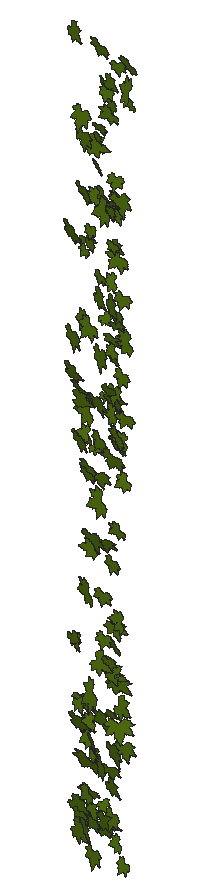
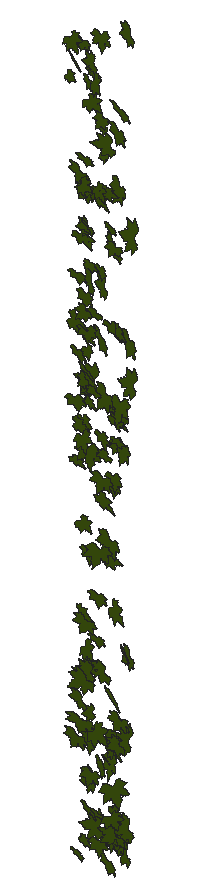
# SketchUp Ruby script. Lengths in inches.
U = 1.inch
M = Sketchup.active_model
def pt(a) = Geom::Point3d.new(a.map { |v| v * U })
def face(e, loops, mat)
  f = e.add_face(loops[0].map { |a| pt(a) })
  loops[1..].each { |l| e.add_face(l.map { |a| pt(a) }).erase! }
  f.material = f.back_material = mat if mat
  f
end
# faces: each face lists its corners as indices into pts; further lists are holes
def faces(e, pts, list, mat = nil) = list.each { |f| face(e, (f[0].is_a?(Array) ? f : [f]).map { |l| l.map { |i| pts[i] } }, mat) }
# xy, xz, yz: faces in a plane at the given z, y or x. An outline is a flat list of corners, or four numbers for a rectangle; further outlines are holes
def ring(l) = l.size == 4 ? [[l[0], l[1]], [l[2], l[1]], [l[2], l[3]], [l[0], l[3]]] : l.each_slice(2).to_a
def flat(e, list, mat, &to3) = list.each { |f| face(e, (f[0].is_a?(Array) ? f : [f]).map { |l| ring(l).map { |u, v| to3.(u, v) } }, mat) }
def xy(e, z, list, mat = nil) = flat(e, list, mat) { |x, y| [x, y, z] }
def xz(e, y, list, mat = nil) = flat(e, list, mat) { |x, z| [x, y, z] }
def yz(e, x, list, mat = nil) = flat(e, list, mat) { |y, z| [x, y, z] }
def lines(e, pts, list) = list.each { |a, b| e.add_line(pt(pts[a]), pt(pts[b])) }
# prism: a flat outline (further loops are holes) pulled along v
def prism(e, loops, v, mat = nil)
  f = face(e, loops, mat); d = Geom::Vector3d.new(v.map { |x| x * U })
  f.pushpull(f.normal.samedirection?(d) ? d.length : -d.length)
end
def box(e, o, s, mat = nil) = prism(e, [[o, [o[0] + s[0], o[1], o[2]], [o[0] + s[0], o[1] + s[1], o[2]], [o[0], o[1] + s[1], o[2]]]], [0, 0, s[2]], mat)
def at(x, y, z, deg = 0) = Geom::Transformation.translation(pt([x, y, z])) * Geom::Transformation.rotation(ORIGIN, Z_AXIS, deg.degrees)
def axes(o, x, y, z) = Geom::Transformation.new([*x, 0, *y, 0, *z, 0, *pt(o).to_a, 1])
def part(name) = M.definitions.add(name)
# library, detail: a bought-in or finely detailed component or shape, given as its bounding box
def library(name, o, s) = part(name).tap { |d| box(d.entities, o, s) }
def detail(e, o, s) = box(e.add_group.entities, o, s)
def put(e, d, t, mat = nil) = e.add_instance(d, t).tap { |i| i.material = mat if mat }
def group(e, t, mat = nil) = e.add_group.tap { |g| g.transformation = t; g.material = mat if mat }.entities
root = M.entities
M.materials.add("[Vegetation Blur 03]").color = [83, 114, 18]
c1 = part("ivy")
xy(c1.entities,0,[[0.782,0,0.786,0,0.787,0.005,0.789,0.009,0.821,0.072,0.875,0.147,1.001,0.272,1.073,0.331,1.137,0.363,1.178,0.379,1.223,0.384,1.272,0.383,1.311,0.374,1.36,0.355,1.399,0.334,1.491,0.285,1.541,0.244,1.583,0.199,1.617,0.15,1.64,0.128,1.662,0.115,1.717,0.105,1.745,0.093,1.784,0.054,1.819,0.057,1.854,0.064,1.882,0.075,1.896,0.074,1.91,0.071,1.937,0.063,1.964,0.053,1.99,0.038,2.016,0.015,2.034,0.002,2.04,0,2.038,0.003,2.036,0.007,2.033,0.038,2.036,0.068,2.045,0.1,2.055,0.116,2.064,0.123,2.077,0.129,2.088,0.129,2.106,0.132,2.118,0.13,2.179,0.132,2.207,0.133,2.225,0.133,2.242,0.138,2.22,0.162,2.207,0.186,2.206,0.213,2.212,0.236,2.228,0.262,2.247,0.274,2.298,0.283,2.355,0.294,2.37,0.296,2.376,0.295,2.377,0.3,2.377,0.303,2.385,0.329,2.411,0.37,2.426,0.392,2.449,0.407,2.511,0.426,2.561,0.444,2.619,0.466,2.589,0.469,2.561,0.476,2.501,0.5,2.449,0.516,2.424,0.523,2.401,0.535,2.377,0.556,2.372,0.568,2.36,0.575,2.268,0.586,2.225,0.592,2.207,0.599,2.194,0.61,2.143,0.65,2.13,0.664,2.122,0.682,2.123,0.7,2.13,0.719,2.148,0.75,2.17,0.781,2.195,0.807,2.221,0.828,2.284,0.874,2.291,0.88,2.288,0.887,2.276,0.9,2.267,0.916,2.265,0.933,2.273,0.967,2.292,1.002,2.313,1.03,2.334,1.054,2.348,1.067,2.358,1.074,2.363,1.076,2.362,1.081,2.35,1.094,2.347,1.11,2.35,1.143,2.359,1.18,2.385,1.254,2.415,1.324,2.448,1.393,2.45,1.4,2.446,1.398,2.44,1.394,2.427,1.383,2.402,1.36,2.376,1.339,2.345,1.324,2.305,1.309,2.282,1.303,2.273,1.306,2.245,1.294,2.212,1.287,2.187,1.291,2.163,1.301,2.142,1.316,2.134,1.327,2.124,1.325,2.09,1.292,2.053,1.259,2.014,1.234,1.973,1.215,1.954,1.21,1.931,1.208,1.909,1.212,1.893,1.22,1.879,1.233,1.872,1.248,1.867,1.281,1.864,1.319,1.821,1.258,1.773,1.197,1.726,1.141,1.698,1.121,1.679,1.116,1.666,1.117,1.647,1.122,1.632,1.129,1.62,1.141,1.617,1.154,1.617,1.219,1.621,1.254,1.623,1.268,1.623,1.281,1.618,1.314,1.606,1.346,1.603,1.375,1.607,1.403,1.603,1.467,1.599,1.499,1.605,1.525,1.614,1.552,1.629,1.577,1.635,1.589,1.629,1.587,1.618,1.582,1.596,1.566,1.581,1.556,1.568,1.552,1.557,1.55,1.545,1.553,1.531,1.562,1.522,1.572,1.504,1.591,1.486,1.611,1.474,1.631,1.457,1.666,1.455,1.684,1.457,1.698,1.452,1.715,1.444,1.728,1.424,1.754,1.419,1.772,1.423,1.786,1.434,1.819,1.444,1.848,1.446,1.855,1.44,1.861,1.43,1.867,1.386,1.904,1.349,1.948,1.326,1.973,1.31,1.995,1.288,2.048,1.284,2.153,1.287,2.254,1.284,2.255,1.282,2.253,1.278,2.247,1.274,2.237,1.266,2.216,1.226,2.125,1.208,2.076,1.184,2.033,1.155,1.984,1.135,1.942,1.111,1.899,1.083,1.861,1.053,1.85,1.059,1.83,1.061,1.809,1.056,1.79,1.049,1.767,1.04,1.749,1.018,1.733,0.994,1.726,0.942,1.734,0.95,1.6875,0.944,1.645,0.932,1.608,0.911,1.585,0.881,1.58,0.854,1.582,0.828,1.588,0.785,1.618,0.773,1.625,0.775,1.614,0.779,1.598,0.796,1.502,0.818,1.402,0.861,1.283,0.882,1.224,0.894,1.174,0.892,1.148,0.886,1.123,0.881,1.107,0.872,1.099,0.849,1.094,0.818,1.092,0.789,1.098,0.762,1.107,0.753,1.113,0.721,1.139,0.698,1.163,0.678,1.194,0.665,1.224,0.628,1.28,0.612,1.312,0.606,1.327,0.606,1.314,0.599,1.282,0.594,1.267,0.581,1.256,0.544,1.245,0.512,1.244,0.473,1.249,0.444,1.256,0.382,1.288,0.339,1.306,0.324,1.316,0.317,1.324,0.309,1.326,0.27,1.314,0.227,1.313,0.185,1.3125,0.152,1.317,0.122,1.328,0.092,1.345,0.073,1.353,0.079,1.338,0.092,1.308,0.117,1.249,0.13,1.215,0.139,1.164,0.147,1.148,0.157,1.136,0.163,1.122,0.174,1.086,0.177,1.067,0.182,1.054,0.186,1.043,0.191,1.038,0.211,1.028,0.237,1.005,0.25,0.974,0.253,0.96,0.25,0.944,0.242,0.914,0.243,0.906,0.249,0.902,0.26,0.894,0.289,0.88,0.307,0.873,0.322,0.862,0.364,0.799,0.403,0.738,0.431,0.709,0.439,0.691,0.441,0.678,0.4375,0.66,0.428,0.645,0.394,0.623,0.303,0.594,0.255,0.581,0.214,0.577,0.179,0.573,0.173,0.568,0.175,0.561,0.167,0.55,0.141,0.523,0.113,0.503,0.077,0.49,0.045,0.486,0.026,0.485,0.019,0.486,0.011,0.483,0,0.471,0.014,0.467,0.044,0.455,0.058,0.447,0.07,0.438,0.097,0.411,0.125,0.394,0.158,0.377,0.174,0.366,0.182,0.359,0.185,0.361,0.242,0.331,0.253,0.316,0.258,0.303,0.262,0.283,0.274,0.278,0.308,0.274,0.341,0.252,0.366,0.226,0.366,0.222,0.37,0.22,0.38,0.221,0.395,0.221,0.425,0.216,0.45,0.207,0.465,0.192,0.473,0.178,0.484,0.15,0.489,0.116,0.483,0.089,0.468,0.058,0.45,0.035,0.435,0.018,0.429,0.011,0.434,0.012,0.438,0.014,0.469,0.019,0.542,0.016,0.581,0.015,0.612,0.027,0.68,0.055,0.696,0.057,0.712,0.052,0.73,0.045,0.741,0.036,0.766,0.014]])
put(root,c1,axes([66.49,173.7,78.62],[0.10022,-0.2222,0.4688],[0.57871,-0.13035,-0.09212],[-0.08191,-1.19279,-0.07727]),"[Vegetation Blur 03]")
put(root,c1,axes([67.61,173.7,82.38],[0.12813,-0.15006,-0.36786],[-0.44192,0.20151,-0.11546],[-0.11482,-0.94298,0.03387]),"[Vegetation Blur 03]")
put(root,c1,axes([66.39,173.7,81.41],[0.62179,-0.3866,0.07255],[0.08725,-0.03824,-0.53009],[-0.18864,-1.29198,-0.00602]),"[Vegetation Blur 03]")
put(root,c1,axes([67.06,173.7,59.03],[0.53027,0.09687,-0.32245],[-0.39653,0.24084,-0.42296],[-0.03295,-1.33931,-0.09938]),"[Vegetation Blur 03]")
put(root,c1,axes([66.45,173.7,64.9],[0.37075,-0.20222,0.27738],[0.33431,-0.13128,-0.31269],[-0.11578,-1.02663,-0.01465]),"[Vegetation Blur 03]")
put(root,c1,axes([66.4375,173.7,96.87],[0.27432,-0.11887,0.39101],[0.46845,-0.2067,-0.22879],[-0.11587,-1.1171,0.00072]),"[Vegetation Blur 03]")
put(root,c1,axes([66.68,173.7,78.54],[0.61753,-0.18671,-0.12394],[-0.12621,0.33022,-0.49708],[-0.12397,-1.26626,-0.11135]),"[Vegetation Blur 03]")
put(root,c1,axes([67.63,173.7,68.17],[0.24952,-0.09563,-0.45788],[-0.54485,0.27669,-0.20686],[-0.14163,-1.23287,-0.01091]),"[Vegetation Blur 03]")
put(root,c1,axes([66.4,173.7,86.14],[0.18149,-0.29755,0.51892],[0.63719,-0.20751,-0.16715],[-0.13848,-1.34475,-0.08903]),"[Vegetation Blur 03]")
put(root,c1,axes([66.8,173.7,64.98],[0.30081,-0.15518,0.1985],[0.21889,-0.23826,-0.25024],[-0.13012,-0.75955,0.03794]),"[Vegetation Blur 03]")
put(root,c1,axes([66.48,173.7,55.85],[0.29611,-0.16504,0.41768],[0.51687,0.01316,-0.24325],[-0.03458,-1.21665,-0.05929]),"[Vegetation Blur 03]")
put(root,c1,axes([66.76,173.7,61.44],[0.29238,-0.00543,0.2431],[0.28843,-0.20948,-0.23179],[-0.07444,-0.83296,0.05671]),"[Vegetation Blur 03]")
put(root,c1,axes([66.71,173.7,75.97],[0.56984,-0.3114,0.00181],[0.01697,0.11385,-0.47886],[-0.15039,-1.16708,-0.04719]),"[Vegetation Blur 03]")
put(root,c1,axes([67.42,173.7,57.23],[0.30579,0.15468,-0.23311],[-0.2938,0.07258,-0.24913],[0.03027,-0.858,-0.0631]),"[Vegetation Blur 03]")
put(root,c1,axes([67.89,173.7,77.98],[0.21628,-0.19716,-0.4852],[-0.59473,0.13393,-0.18514],[-0.09444,-1.29492,0.05473]),"[Vegetation Blur 03]")
put(root,c1,axes([66.71,173.7,61.84],[0.46672,-0.03992,0.15461],[0.18977,0.01161,-0.3811],[-0.01585,-1.03645,-0.01022]),"[Vegetation Blur 03]")
put(root,c1,axes([66.79,173.7,55.93],[0.51714,-0.23527,0.06533],[0.0842,0.02179,-0.43163],[-0.1113,-1.07662,-0.02301]),"[Vegetation Blur 03]")
put(root,c1,axes([67.9,173.7,76.375],[0.04403,-0.12753,-0.27738],[-0.34532,-0.03734,-0.03381],[0.01033,-0.70424,0.05202]),"[Vegetation Blur 03]")
put(root,c1,axes([67.375,173.7,85.94],[0.27643,-0.11245,-0.0959],[-0.1208,-0.01738,-0.22873],[-0.04691,-0.61786,0.02389]),"[Vegetation Blur 03]")
put(root,c1,axes([66.8125,173.7,60.14],[0.09309,-0.2572,0.47512],[0.59358,-0.05541,-0.08218],[-0.0469,-1.21192,-0.09707]),"[Vegetation Blur 03]")
put(root,c1,axes([66.6875,173.7,54.4],[0.19741,-0.09695,0.50499],[0.60705,-0.24693,-0.16553],[-0.12869,-1.3135,-0.00615]),"[Vegetation Blur 03]")
put(root,c1,axes([66.87,173.7,77.11],[0.08822,-0.12322,0.46198],[0.56917,0.00464,-0.0722],[-0.00698,-1.17889,-0.04857]),"[Vegetation Blur 03]")
put(root,c1,axes([67.09,173.7,86.17],[0.33638,0.01493,0.11781],[0.14294,0.07701,-0.27338],[0.02139,-0.74929,-0.02575]),"[Vegetation Blur 03]")
put(root,c1,axes([67.55,173.7,57.4],[0.34978,-0.17504,-0.23097],[-0.28247,0.06704,-0.29293],[-0.08681,-0.92345,0.02252]),"[Vegetation Blur 03]")
put(root,c1,axes([66.95,173.7,60.24],[0.25126,-0.00237,0.3092],[0.37875,0.02524,-0.20497],[0.00958,-0.93516,-0.00632]),"[Vegetation Blur 03]")
put(root,c1,axes([67.3,173.7,74.54],[0.44154,-0.10792,-0.13293],[-0.15664,0.11844,-0.36167],[-0.06888,-0.96117,-0.02964]),"[Vegetation Blur 03]")
put(root,c1,axes([67.32,173.7,74.13],[0.39751,-0.09835,-0.09675],[-0.112,0.11608,-0.32505],[-0.0616,-0.84567,-0.03337]),"[Vegetation Blur 03]")
put(root,c1,axes([66.93,173.7,93.25],[0.5878,-0.24093,0.03931],[0.02588,-0.23212,-0.48155],[-0.12393,-1.19122,0.08588]),"[Vegetation Blur 03]")
put(root,c1,axes([68.2,173.7,70.44],[0.06394,-0.03491,-0.38067],[-0.46672,-0.01334,-0.05203],[0.00412,-0.96871,0.01444]),"[Vegetation Blur 03]")
put(root,c1,axes([67.71,173.7,60.375],[0.28202,-0.18926,-0.22565],[-0.28437,-0.00619,-0.23592],[-0.06351,-0.81269,0.05435]),"[Vegetation Blur 03]")
put(root,c1,axes([67.47,173.7,75.98],[0.28723,-0.15203,-0.02555],[-0.02588,0.0511,-0.24162],[-0.07595,-0.59236,-0.01429]),"[Vegetation Blur 03]")
put(root,c1,axes([66.9375,173.7,89.15],[0.5598,-0.34639,0.09978],[0.13771,0.07562,-0.47332],[-0.15594,-1.17668,-0.05979]),"[Vegetation Blur 03]")
put(root,c1,axes([67,173.7,92.08],[0.56579,-0.26175,0.06944],[0.08066,-0.05979,-0.47321],[-0.13005,-1.17586,0.0086]),"[Vegetation Blur 03]")
put(root,c1,axes([68.08,173.7,61.22],[0.11929,-0.10597,-0.2818],[-0.34889,-0.06251,-0.09467],[0.01224,-0.74914,0.04776]),"[Vegetation Blur 03]")
put(root,c1,axes([67.54,173.7,82.3],[0.50454,-0.20666,-0.19788],[-0.2502,-0.0525,-0.4163],[-0.0792,-1.15072,0.05453]),"[Vegetation Blur 03]")
put(root,c1,axes([66.85,173.7,55.51],[0.43162,0.02667,0.37239],[0.45622,0.01814,-0.35241],[0.01531,-1.29236,0.00274]),"[Vegetation Blur 03]")
put(root,c1,axes([67.5,173.7,59.9],[0.51252,-0.27009,-0.18144],[-0.18784,0.30748,-0.42542],[-0.17711,-1.10772,-0.07385]),"[Vegetation Blur 03]")
put(root,c1,axes([67.56,173.7,56.04],[0.4822,-0.17189,-0.16775],[-0.19534,0.15084,-0.39833],[-0.10519,-1.06807,-0.02926]),"[Vegetation Blur 03]")
put(root,c1,axes([68.39,173.7,89.16],[0.05825,-0.05857,-0.32384],[-0.39732,-0.0501,-0.04618],[0.02002,-0.82377,0.02584]),"[Vegetation Blur 03]")
put(root,c1,axes([67.02,173.7,55.04],[0.3696,-0.27711,0.38105],[0.45779,-0.2062,-0.31935],[-0.16294,-1.2079,-0.0329]),"[Vegetation Blur 03]")
put(root,c1,axes([67.58,173.7,87.01],[0.33002,-0.10362,0.05882],[0.06392,-0.11285,-0.27012],[-0.06037,-0.68589,0.03556]),"[Vegetation Blur 03]")
put(root,c1,axes([67.53,173.7,86.21],[0.29872,-0.15455,0.15212],[0.18312,-0.07365,-0.25129],[-0.08276,-0.72081,-0.00694]),"[Vegetation Blur 03]")
put(root,c1,axes([67.96,173.7,63.21],[0.5074,-0.4678,-0.2898],[-0.37384,0.02954,-0.44347],[-0.19497,-1.27408,0.09613]),"[Vegetation Blur 03]")
put(root,c1,axes([67.71,173.7,75.02],[0.11399,0.08931,0.26369],[0.32563,0.00233,-0.09389],[0.01551,-0.70503,0.03309]),"[Vegetation Blur 03]")
put(root,c1,axes([67.25,173.7,70.8],[0.63866,-0.23189,0.12864],[0.16822,0.10928,-0.52532],[-0.09614,-1.34925,-0.06466]),"[Vegetation Blur 03]")
put(root,c1,axes([68.54,173.7,61.51],[0.24902,0.09318,-0.40988],[-0.50306,0.12516,-0.1991],[-0.03467,-1.14673,-0.05504]),"[Vegetation Blur 03]")
put(root,c1,axes([67.55,173.7,90.76],[0.09049,0.02962,0.47011],[0.57571,0.04471,-0.07426],[0.0237,-1.19903,0.00884]),"[Vegetation Blur 03]")
put(root,c1,axes([67.83,173.7,59.24],[0.27201,-0.08351,0.1346],[0.14493,-0.22002,-0.21655],[-0.08857,-0.61651,0.05905]),"[Vegetation Blur 03]")
put(root,c1,axes([68.66,173.7,94.97],[0.14161,0.02749,-0.37414],[-0.43235,0.33737,-0.1051],[-0.153,-0.92792,-0.0493]),"[Vegetation Blur 03]")
put(root,c1,axes([68.43,173.7,73.4375],[0.39569,-0.25539,-0.40505],[-0.50198,0.05522,-0.33211],[-0.09868,-1.305,0.06522]),"[Vegetation Blur 03]")
put(root,c1,axes([67.73,173.7,59.69],[0.16819,-0.22664,0.32974],[0.39401,-0.21788,-0.15742],[-0.14187,-0.87383,-0.04627]),"[Vegetation Blur 03]")
put(root,c1,axes([67.64,173.7,54.19],[0.53858,-0.252,0.05397],[0.05479,-0.1161,-0.44944],[-0.12794,-1.11057,0.03474]),"[Vegetation Blur 03]")
put(root,c1,axes([67.92,173.7,97.125],[0.51011,-0.11701,-0.13612],[-0.15838,0.15628,-0.41647],[-0.07724,-1.09327,-0.04497]),"[Vegetation Blur 03]")
put(root,c1,axes([68.43,173.7,89.34],[0.31562,-0.0779,-0.30416],[-0.3657,0.1532,-0.25894],[-0.08116,-0.99323,-0.01608]),"[Vegetation Blur 03]")
put(root,c1,axes([68.03,173.7,55.54],[0.43132,0.00683,-0.12215],[-0.14822,0.15148,-0.34728],[-0.02104,-0.9272,-0.05763]),"[Vegetation Blur 03]")
put(root,c1,axes([67.72,173.7,70.54],[0.54712,0.06533,0.00829],[0.00324,0.23778,-0.43729],[0.03318,-1.10066,-0.09398]),"[Vegetation Blur 03]")
put(root,c1,axes([67.68,173.7,74.03],[0.51598,-0.04836,0.08245],[0.10256,0.07999,-0.4201],[-0.01553,-1.07898,-0.03484]),"[Vegetation Blur 03]")
put(root,c1,axes([68.11,173.7,76.36],[0.44792,-0.20906,-0.13241],[-0.16237,0.03502,-0.37455],[-0.10139,-0.9797,0.01487]),"[Vegetation Blur 03]")
put(root,c1,axes([67.91,173.7,92.5],[0.35213,-0.1038,0.09821],[0.12718,0.11373,-0.28482],[-0.02917,-0.75727,-0.05624]),"[Vegetation Blur 03]")
put(root,c1,axes([68.21,173.7,84.87],[0.35103,-0.1488,-0.07514],[-0.0909,0.03087,-0.29249],[-0.07377,-0.74614,0.00288]),"[Vegetation Blur 03]")
put(root,c1,axes([68.04,173.7,91.92],[0.22551,-0.17157,0.19026],[0.23404,-0.06401,-0.19384],[-0.08079,-0.66437,-0.03046]),"[Vegetation Blur 03]")
put(root,c1,axes([68.7,173.7,88.93],[0.36429,-0.26691,-0.39719],[-0.49048,0.09297,-0.30946],[-0.1145,-1.24751,0.06192]),"[Vegetation Blur 03]")
put(root,c1,axes([67.75,173.7,63.54],[0.19537,0.05525,0.44525],[0.54604,-0.05051,-0.1586],[-0.01409,-1.19141,0.02737]),"[Vegetation Blur 03]")
put(root,c1,axes([67.98,173.7,90.58],[0.31604,-0.28517,0.16056],[0.20748,-0.01555,-0.27638],[-0.12189,-0.7659,-0.05417]),"[Vegetation Blur 03]")
put(root,c1,axes([67.64,173.7,78.11],[0.57292,-0.29787,0.17247],[0.22282,0.05394,-0.47834],[-0.12636,-1.25544,-0.06147]),"[Vegetation Blur 03]")
put(root,c1,axes([68.13,173.7,67.97],[0.45876,-0.06676,-0.02085],[-0.02631,-0.02088,-0.37522],[-0.03182,-0.94526,0.00976]),"[Vegetation Blur 03]")
put(root,c1,axes([68.23,173.7,56.47],[0.21181,0.06558,0.16158],[0.19963,-0.12494,-0.16633],[-0.01894,-0.58339,0.05378]),"[Vegetation Blur 03]")
put(root,c1,axes([68.875,173.7,93.78],[0.26725,0.04128,-0.32232],[-0.39537,0.00799,-0.21819],[0.00802,-0.98126,-0.01534]),"[Vegetation Blur 03]")
put(root,c1,axes([68.28,173.7,65.7],[0.40879,-0.06868,-0.00639],[-0.01176,-0.09983,-0.33231],[-0.0322,-0.83542,0.04024]),"[Vegetation Blur 03]")
put(root,c1,axes([68.3,173.7,59.26],[0.4884,-0.38994,-0.09349],[-0.11293,0.05241,-0.42733],[-0.19047,-1.03097,0.01363]),"[Vegetation Blur 03]")
put(root,c1,axes([68.27,173.7,82.23],[0.21448,0.07418,0.20841],[0.25788,-0.06923,-0.1729],[-0.00284,-0.68276,0.04017]),"[Vegetation Blur 03]")
put(root,c1,axes([68.05,173.7,83.25],[0.21062,-0.15839,0.41958],[0.49728,-0.27124,-0.18238],[-0.15148,-1.11064,-0.0153]),"[Vegetation Blur 03]")
put(root,c1,axes([69.09,173.7,65.58],[0.21131,0.04206,-0.34485],[-0.41038,0.25638,-0.16258],[-0.10272,-0.93777,-0.05992]),"[Vegetation Blur 03]")
put(root,c1,axes([68.33,173.7,78.15],[0.18344,0.08958,0.24161],[0.29922,-0.05038,-0.14838],[0.0019,-0.7149,0.04073]),"[Vegetation Blur 03]")
put(root,c1,axes([68.07,173.7,80.88],[0.58162,-0.37165,0.13863],[0.15197,-0.16988,-0.49633],[-0.1959,-1.23523,0.02655]),"[Vegetation Blur 03]")
put(root,c1,axes([68.5,173.7,94.72],[0.38042,-0.08348,0.02066],[0.01844,-0.12918,-0.30833],[-0.04412,-0.77385,0.04924]),"[Vegetation Blur 03]")
put(root,c1,axes([68.41,173.7,58.68],[0.44484,-0.01751,0.04002],[0.04967,0.10203,-0.36079],[-0.00297,-0.91526,-0.04099]),"[Vegetation Blur 03]")
put(root,c1,axes([68.47,173.7,64.36],[0.36338,-0.06137,0.0857],[0.10665,0.03955,-0.29676],[-0.02326,-0.77736,-0.02186]),"[Vegetation Blur 03]")
put(root,c1,axes([68.52,173.7,75.66],[0.62172,-0.07982,-0.18766],[-0.22411,0.16779,-0.50577],[-0.06444,-1.35373,-0.05162]),"[Vegetation Blur 03]")
put(root,c1,axes([69.01,173.7,80.71],[0.25042,-0.03463,-0.18206],[-0.21423,0.16131,-0.2011],[-0.06442,-0.671,-0.03895]),"[Vegetation Blur 03]")
put(root,c1,axes([69.46,173.7,89.26],[0.07231,0.11382,-0.30015],[-0.37128,0.06711,-0.05557],[-0.02172,-0.76837,-0.04931]),"[Vegetation Blur 03]")
put(root,c1,axes([69.36,173.7,85.02],[0.14335,-0.13764,-0.29117],[-0.36286,-0.03379,-0.11648],[-0.00945,-0.79049,0.05568]),"[Vegetation Blur 03]")
put(root,c1,axes([69.33,173.7,78.09],[0.18991,-0.19032,-0.31472],[-0.38839,0.08836,-0.16451],[-0.08006,-0.88012,0.05154]),"[Vegetation Blur 03]")
put(root,c1,axes([68.33,173.7,55.26],[0.11966,-0.19885,0.48664],[0.60405,0.04067,-0.09632],[0.00062,-1.25082,-0.0805]),"[Vegetation Blur 03]")
put(root,c1,axes([68.69,173.7,81.65],[0.43667,-0.00599,-0.05285],[-0.0643,0.07555,-0.35518],[-0.00825,-0.90526,-0.02929]),"[Vegetation Blur 03]")
put(root,c1,axes([69.19,173.7,81.25],[0.22039,-0.10268,-0.20891],[-0.2592,-0.01,-0.18136],[-0.02883,-0.69502,0.03347]),"[Vegetation Blur 03]")
put(root,c1,axes([69.1,173.7,76.3],[0.37381,-0.01776,-0.27785],[-0.3272,0.26974,-0.29592],[-0.09444,-1.00486,-0.07453]),"[Vegetation Blur 03]")
put(root,c1,axes([68.79,173.7,61.36],[0.12453,-0.12682,0.21988],[0.27637,0.0612,-0.0987],[0.00185,-0.60769,-0.05583]),"[Vegetation Blur 03]")
put(root,c1,axes([69.36,173.7,71.83],[0.24891,0.01709,-0.28911],[-0.35411,0.04401,-0.20266],[-0.01273,-0.88984,-0.01558]),"[Vegetation Blur 03]")
put(root,c1,axes([68.63,173.7,94.71],[0.15082,-0.08194,0.36497],[0.44384,-0.11913,-0.12637],[-0.06768,-0.96384,-0.01541]),"[Vegetation Blur 03]")
put(root,c1,axes([68.81,173.7,69.99],[0.46442,-0.17928,-0.04706],[-0.05947,-0.00913,-0.38545],[-0.0859,-0.96299,0.01241]),"[Vegetation Blur 03]")
put(root,c1,axes([68.76,173.7,88.34],[0.3125,-0.15896,0.12959],[0.15654,-0.05797,-0.26261],[-0.08171,-0.71898,-0.00748]),"[Vegetation Blur 03]")
put(root,c1,axes([69.8125,173.7,67.13],[0.07751,-0.08641,-0.39879],[-0.48715,0.10409,-0.06661],[-0.05668,-1.01274,0.02718]),"[Vegetation Blur 03]")
put(root,c1,axes([68.84,173.7,94.1],[0.3345,-0.16348,0.07359],[0.08724,-0.0471,-0.28058],[-0.08265,-0.71135,0.00167]),"[Vegetation Blur 03]")
put(root,c1,axes([68.8125,173.7,86.55],[0.32611,-0.0735,0.11387],[0.13621,-0.07341,-0.2673],[-0.04678,-0.72621,0.01549]),"[Vegetation Blur 03]")
put(root,c1,axes([69.52,173.7,55.31],[0.2031,-0.14404,-0.26055],[-0.32267,0.0347,-0.17055],[-0.052,-0.77785,0.04064]),"[Vegetation Blur 03]")
put(root,c1,axes([69.16,173.7,76.97],[0.45681,-0.21004,-0.23078],[-0.27305,0.15298,-0.3819],[-0.12578,-1.09491,-0.00909]),"[Vegetation Blur 03]")
put(root,c1,axes([68.73,173.7,63.1875],[0.0827,0.01826,0.45445],[0.55686,-0.01784,-0.06738],[-0.00727,-1.15829,0.0082]),"[Vegetation Blur 03]")
put(root,c1,axes([68.61,173.7,66.28],[0.50405,-0.0121,0.1413],[0.17315,0.00073,-0.4114],[-0.00545,-1.09673,-0.00183]),"[Vegetation Blur 03]")
put(root,c1,axes([68.82,173.7,88.54],[0.28631,-0.17737,0.19402],[0.25002,0.08801,-0.2331],[-0.03783,-0.76071,-0.07221]),"[Vegetation Blur 03]")
put(root,c1,axes([68.91,173.7,83.22],[0.46399,-0.15608,-0.0301],[-0.03246,0.06122,-0.3832],[-0.07784,-0.95586,-0.01963]),"[Vegetation Blur 03]")
put(root,c1,axes([68.85,173.7,82.17],[0.30561,-0.04373,0.17256],[0.21196,0.11676,-0.24539],[0.01507,-0.75575,-0.0479]),"[Vegetation Blur 03]")
put(root,c1,axes([68.87,173.7,56.6],[0.49081,-0.25055,0.00673],[-0.00728,-0.13032,-0.40947],[-0.12182,-1.0017,0.05159]),"[Vegetation Blur 03]")
put(root,c1,axes([68.96,173.7,90.21],[0.40348,-0.0468,0.02113],[0.02171,-0.14086,-0.32526],[-0.02676,-0.81998,0.05467]),"[Vegetation Blur 03]")
put(root,c1,axes([69.25,173.7,86.51],[0.49046,-0.12487,-0.25125],[-0.31171,-0.05916,-0.40067],[-0.03597,-1.19015,0.04628]),"[Vegetation Blur 03]")
put(root,c1,axes([68.75,173.7,78.02],[0.0827,-0.23642,0.52033],[0.64705,-0.03418,-0.07095],[-0.03151,-1.3225,-0.09118]),"[Vegetation Blur 03]")
put(root,c1,axes([68.72,173.7,57.65],[0.28606,-0.20547,0.36321],[0.44363,-0.1257,-0.24391],[-0.10592,-1.08138,-0.04066]),"[Vegetation Blur 03]")
put(root,c1,axes([69.01,173.7,96.17],[0.38022,-0.03036,0.06928],[0.08439,-0.02832,-0.31043],[-0.01739,-0.80118,0.00835]),"[Vegetation Blur 03]")
put(root,c1,axes([68.91,173.7,79.01],[0.44605,-0.17185,0.11357],[0.12178,-0.19918,-0.36599],[-0.10728,-0.94065,0.05675]),"[Vegetation Blur 03]")
put(root,c1,axes([70.03,173.7,76.72],[0.06632,-0.08264,-0.34848],[-0.42857,0.02082,-0.0551],[-0.0162,-0.88896,0.0311]),"[Vegetation Blur 03]")
put(root,c1,axes([69.02,173.7,78.4],[0.3929,-0.21833,0.06927],[0.09371,0.04854,-0.33],[-0.09838,-0.82573,-0.03771]),"[Vegetation Blur 03]")
put(root,c1,axes([68.63,173.7,62.95],[0.37722,-0.01424,0.37521],[0.45787,0.12358,-0.30587],[0.04206,-1.2175,-0.03543]),"[Vegetation Blur 03]")
put(root,c1,axes([68.88,173.7,88.21],[0.36838,-0.06003,0.20905],[0.25298,-0.09287,-0.30112],[-0.04965,-0.91861,0.01678]),"[Vegetation Blur 03]")
put(root,c1,axes([69.1,173.7,78.58],[0.28308,-0.16005,0.12566],[0.16212,0.03888,-0.23548],[-0.05892,-0.66197,-0.04421]),"[Vegetation Blur 03]")
put(root,c1,axes([69.03,173.7,86.23],[0.16779,-0.0883,0.30239],[0.37001,-0.06611,-0.13979],[-0.04708,-0.83437,-0.02093]),"[Vegetation Blur 03]")
put(root,c1,axes([68.78,173.7,83.1875],[0.25712,-0.18798,0.42224],[0.4923,-0.32764,-0.22263],[-0.18343,-1.14283,-0.00563]),"[Vegetation Blur 03]")
put(root,c1,axes([68.66,173.7,61.12],[0.61342,0.08443,0.16311],[0.20359,-0.16924,-0.49623],[0.01316,-1.31678,0.07424]),"[Vegetation Blur 03]")
put(root,c1,axes([70.18,173.7,82.22],[0.15478,-0.07462,-0.45486],[-0.55676,0.07347,-0.12809],[-0.04416,-1.18802,0.02065]),"[Vegetation Blur 03]")
put(root,c1,axes([69.79,173.7,96.67],[0.32569,0.04627,-0.29452],[-0.35796,0.18221,-0.25916],[-0.05099,-0.98359,-0.06186]),"[Vegetation Blur 03]")
put(root,c1,axes([68.73,173.7,59.98],[0.55958,-0.3731,0.26041],[0.3198,-0.09162,-0.47837],[-0.18004,-1.32239,-0.04033]),"[Vegetation Blur 03]")
put(root,c1,axes([69.44,173.7,77.87],[0.44969,-0.01244,-0.10758],[-0.13185,-0.00591,-0.36702],[-0.00499,-0.96429,0.00364]),"[Vegetation Blur 03]")
put(root,c1,axes([70.39,173.7,95.54],[0.07293,-0.28065,-0.423],[-0.50755,0.30955,-0.09059],[-0.17213,-1.03162,0.0879]),"[Vegetation Blur 03]")
put(root,c1,axes([69.38,173.7,84.12],[0.43256,-0.06671,-0.01604],[-0.02325,-0.10108,-0.35159],[-0.02994,-0.88528,0.04135]),"[Vegetation Blur 03]")
put(root,c1,axes([69.875,173.7,74.7],[0.28967,-0.12811,-0.2275],[-0.2852,-0.08534,-0.23432],[-0.01552,-0.82284,0.05972]),"[Vegetation Blur 03]")
put(root,c1,axes([69.18,173.7,61.63],[0.13579,0.06981,0.42324],[0.51409,-0.17958,-0.1052],[-0.07611,-1.08841,0.0445]),"[Vegetation Blur 03]")
put(root,c1,axes([69.43,173.7,80.09],[0.442,-0.16404,-0.03453],[-0.05057,-0.08968,-0.36412],[-0.07475,-0.90929,0.04214]),"[Vegetation Blur 03]")
put(root,c1,axes([68.96,173.7,89.1],[0.56013,-0.13091,0.22183],[0.26451,-0.15182,-0.45897],[-0.08921,-1.27215,0.03195]),"[Vegetation Blur 03]")
put(root,c1,axes([69.6875,173.7,54.27],[0.36884,-0.18268,-0.08765],[-0.12074,-0.10682,-0.30338],[-0.06956,-0.78327,0.06182]),"[Vegetation Blur 03]")
put(root,c1,axes([69.18,173.7,60.09],[0.51003,-0.05161,0.17077],[0.20792,-0.06034,-0.4165],[-0.03431,-1.13281,0.01441]),"[Vegetation Blur 03]")
put(root,c1,axes([70.26,173.7,94.51],[0.10604,0.023,-0.23018],[-0.28135,0.05824,-0.08542],[-0.02259,-0.61729,-0.01663]),"[Vegetation Blur 03]")
